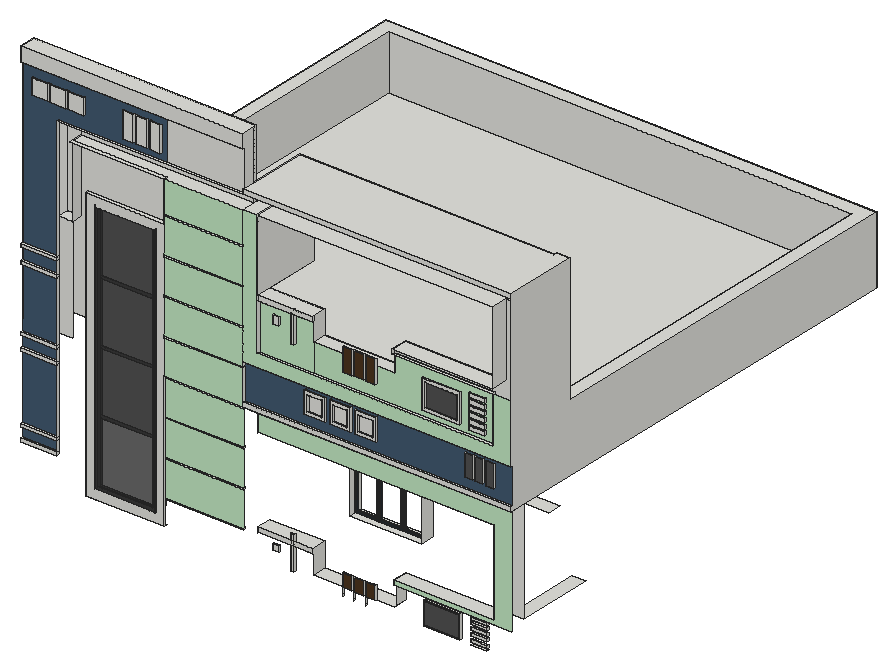
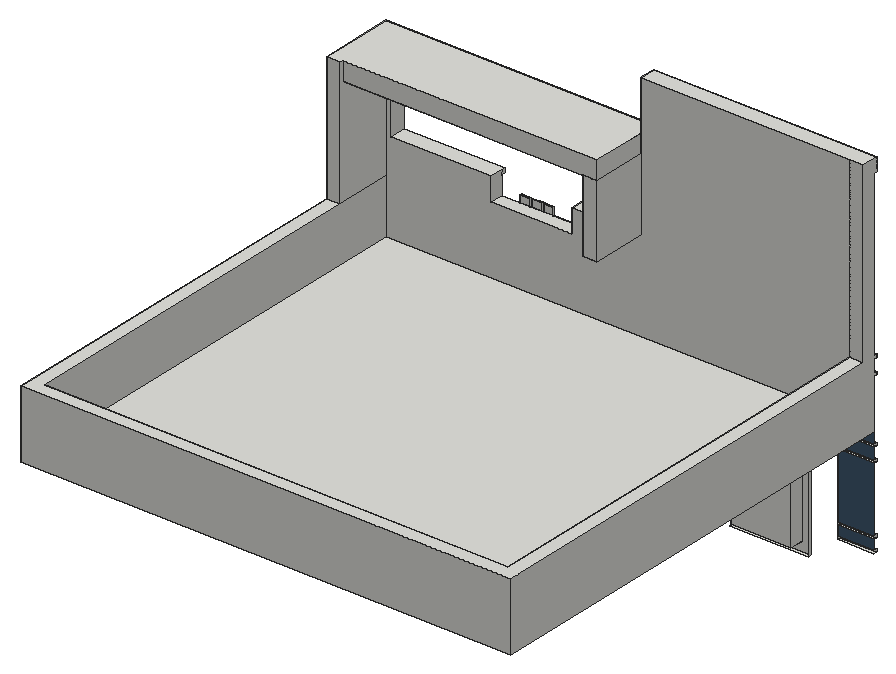
# SketchUp Ruby script. Lengths in inches.
U = 1.inch
M = Sketchup.active_model
def pt(a) = Geom::Point3d.new(a.map { |v| v * U })
def face(e, loops, mat)
  f = e.add_face(loops[0].map { |a| pt(a) })
  loops[1..].each { |l| e.add_face(l.map { |a| pt(a) }).erase! }
  f.material = f.back_material = mat if mat
  f
end
# faces: each face lists its corners as indices into pts; further lists are holes
def faces(e, pts, list, mat = nil) = list.each { |f| face(e, (f[0].is_a?(Array) ? f : [f]).map { |l| l.map { |i| pts[i] } }, mat) }
# xy, xz, yz: faces in a plane at the given z, y or x. An outline is a flat list of corners, or four numbers for a rectangle; further outlines are holes
def ring(l) = l.size == 4 ? [[l[0], l[1]], [l[2], l[1]], [l[2], l[3]], [l[0], l[3]]] : l.each_slice(2).to_a
def flat(e, list, mat, &to3) = list.each { |f| face(e, (f[0].is_a?(Array) ? f : [f]).map { |l| ring(l).map { |u, v| to3.(u, v) } }, mat) }
def xy(e, z, list, mat = nil) = flat(e, list, mat) { |x, y| [x, y, z] }
def xz(e, y, list, mat = nil) = flat(e, list, mat) { |x, z| [x, y, z] }
def yz(e, x, list, mat = nil) = flat(e, list, mat) { |y, z| [x, y, z] }
def lines(e, pts, list) = list.each { |a, b| e.add_line(pt(pts[a]), pt(pts[b])) }
# prism: a flat outline (further loops are holes) pulled along v
def prism(e, loops, v, mat = nil)
  f = face(e, loops, mat); d = Geom::Vector3d.new(v.map { |x| x * U })
  f.pushpull(f.normal.samedirection?(d) ? d.length : -d.length)
end
def box(e, o, s, mat = nil) = prism(e, [[o, [o[0] + s[0], o[1], o[2]], [o[0] + s[0], o[1] + s[1], o[2]], [o[0], o[1] + s[1], o[2]]]], [0, 0, s[2]], mat)
def at(x, y, z, deg = 0) = Geom::Transformation.translation(pt([x, y, z])) * Geom::Transformation.rotation(ORIGIN, Z_AXIS, deg.degrees)
def axes(o, x, y, z) = Geom::Transformation.new([*x, 0, *y, 0, *z, 0, *pt(o).to_a, 1])
def part(name) = M.definitions.add(name)
# library, detail: a bought-in or finely detailed component or shape, given as its bounding box
def library(name, o, s) = part(name).tap { |d| box(d.entities, o, s) }
def detail(e, o, s) = box(e.add_group.entities, o, s)
def put(e, d, t, mat = nil) = e.add_instance(d, t).tap { |i| i.material = mat if mat }
def group(e, t, mat = nil) = e.add_group.tap { |g| g.transformation = t; g.material = mat if mat }.entities
root = M.entities
M.materials.add("Teddy_SkinShadow ").color = [76, 52, 30]
M.materials.add("Wine2").color = [0, 0, 0]
M.materials["Wine2"].alpha = 0
M.materials.add("[0111_SlateGray]").color = [66, 89, 112]
M.materials.add("[0116_Lavender]").color = [195, 232, 195]
M.materials.add("[0130_Gainsboro]").color = [39, 45, 50]
M.materials.add("[0134_DimGray]").color = [105, 105, 105]
M.materials.add("[0135_DarkGray]1").color = [81, 81, 81]
M.materials.add("[0136_Charcoal]").color = [35, 35, 35]
M.materials.add("[Color M07]").color = [58, 58, 58]
c1 = part("Framed glazing panel")
xy(c1.entities,0,[[0,-0.98,43.07,0],[0,0,43.07,1.4]],"[0130_Gainsboro]")
xy(c1.entities,0.3,[[0.3,-1.43,42.77,-0.98]],"[0130_Gainsboro]")
xy(c1.entities,2.95,[[2.95,-1.43,40.12,-0.63],[2.95,-0.63,40.12,0],[2.95,0,40.12,0.64],[2.95,0.64,40.12,1.4]],"[0130_Gainsboro]")
xy(c1.entities,3.54,[[3.54,-0.63,39.53,0],[3.54,0,39.53,0.64]],"[0130_Gainsboro]")
xy(c1.entities,111.8125,[[3.54,-0.63,39.53,0],[3.54,0,39.53,0.64]],"[0130_Gainsboro]")
xy(c1.entities,112.4,[[2.95,-1.43,40.12,-0.63],[2.95,-0.63,40.12,0],[2.95,0,40.12,0.64],[2.95,0.64,40.12,1.4]],"[0130_Gainsboro]")
xy(c1.entities,115.05,[[0.3,-1.43,42.77,-0.98]],"[0130_Gainsboro]")
xy(c1.entities,115.35,[[0,-0.98,43.07,0],[0,0,43.07,1.4]],"[0130_Gainsboro]")
xz(c1.entities,-1.43,[[[0.3,0.3,42.77,115.05],[2.95,2.95,40.12,112.4]]],"[0130_Gainsboro]")
xz(c1.entities,-0.98,[[[0,0,43.07,115.35],[0.3,0.3,42.77,115.05]]],"[0130_Gainsboro]")
xz(c1.entities,-0.63,[[[2.95,2.95,40.12,112.4],[3.54,3.54,39.53,111.8125]]],"[0130_Gainsboro]")
xz(c1.entities,0,[[3.54,3.54,39.53,111.8125]],"Wine2")
xz(c1.entities,0,[[[0,0,43.07,115.35],[2.95,2.95,40.12,112.4]],[[2.95,2.95,40.12,112.4],[3.54,3.54,39.53,111.8125]]],"[0130_Gainsboro]")
xz(c1.entities,0.64,[[[2.95,2.95,40.12,112.4],[3.54,3.54,39.53,111.8125]]],"[0130_Gainsboro]")
xz(c1.entities,1.4,[[[0,0,43.07,115.35],[2.95,2.95,40.12,112.4]]],"[0130_Gainsboro]")
yz(c1.entities,0,[[-0.98,0,0,115.35],[0,0,1.4,115.35]],"[0130_Gainsboro]")
yz(c1.entities,0.3,[[-1.43,0.3,-0.98,115.05]],"[0130_Gainsboro]")
yz(c1.entities,2.95,[[-1.43,2.95,-0.63,112.4],[-0.63,2.95,0,112.4],[0,2.95,0.64,112.4],[0.64,2.95,1.4,112.4]],"[0130_Gainsboro]")
yz(c1.entities,3.54,[[-0.63,3.54,0,111.8125],[0,3.54,0.64,111.8125]],"[0130_Gainsboro]")
yz(c1.entities,39.53,[[-0.63,3.54,0,111.8125],[0,3.54,0.64,111.8125]],"[0130_Gainsboro]")
yz(c1.entities,40.12,[[-1.43,2.95,-0.63,112.4],[-0.63,2.95,0,112.4],[0,2.95,0.64,112.4],[0.64,2.95,1.4,112.4]],"[0130_Gainsboro]")
yz(c1.entities,42.77,[[-1.43,0.3,-0.98,115.05]],"[0130_Gainsboro]")
yz(c1.entities,43.07,[[-0.98,0,0,115.35],[0,0,1.4,115.35]],"[0130_Gainsboro]")
c2 = part("Glazed window assembly")
put(c2.entities,c1,axes([90.57,1.43,0],[1.05148,0,0],[0,1,0],[0,0,1]))
put(c2.entities,c1,axes([0,1.43,0],[1.05148,0,0],[0,1,0],[0,0,1]))
put(c2.entities,c1,axes([45.29,1.43,0],[1.05148,0,0],[0,1,0],[0,0,1]))
c3 = part("window")
g1 = group(c3.entities,at(0,0,0))
g2 = group(g1,at(1.57,1.57,27.56))
yz(g2,0,[[0,0,20.47,25.2]],"[0135_DarkGray]1")
g3 = group(g1,at(1.57,1.57,1.57))
yz(g3,0,[[0,0,20.47,25.2]],"[0134_DimGray]")
g4 = group(g1,at(1.57,1.57,53.54),"[0135_DarkGray]1")
yz(g4,0,[[0,0,20.47,25.2]],"[0135_DarkGray]1")
g5 = group(g1,at(1.57,1.57,79.53))
yz(g5,0,[[0,0,20.47,25.2]],"[0135_DarkGray]1")
g6 = group(g1,at(0,0,0))
xy(g6,0,[[0,0,2.76,23.62]],"[Color M07]")
xy(g6,1.18,[[0,1.18,1.18,22.44],[1.97,1.18,2.76,22.44]],"[Color M07]")
xy(g6,1.57,[[1.18,1.57,1.97,22.05]],"[Color M07]")
xy(g6,26.77,[[1.18,1.57,1.97,22.05]],"[Color M07]")
xy(g6,27.56,[[1.18,1.57,1.97,22.05]],"[Color M07]")
xy(g6,52.76,[[1.18,1.57,1.97,22.05]],"[Color M07]")
xy(g6,53.54,[[1.18,1.57,1.97,22.05]],"[Color M07]")
xy(g6,78.74,[[1.18,1.57,1.97,22.05]],"[Color M07]")
xy(g6,79.53,[[1.18,1.57,1.97,22.05]],"[Color M07]")
xy(g6,104.72,[[1.18,1.57,1.97,22.05]],"[Color M07]")
xy(g6,105.12,[[0,1.18,1.18,22.44],[1.97,1.18,2.76,22.44]],"[Color M07]")
xy(g6,106.3,[[0,0,2.76,23.62]],"[Color M07]")
xz(g6,0,[[0,0,2.76,106.3]],"[Color M07]")
xz(g6,1.18,[[0,1.18,1.18,105.12],[1.97,1.18,2.76,105.12]],"[Color M07]")
xz(g6,1.57,[[1.18,1.57,1.97,26.77],[1.18,27.56,1.97,52.76],[1.18,53.54,1.97,78.74],[1.18,79.53,1.97,104.72]],"[Color M07]")
xz(g6,22.05,[[1.18,1.57,1.97,26.77],[1.18,27.56,1.97,52.76],[1.18,53.54,1.97,78.74],[1.18,79.53,1.97,104.72]],"[Color M07]")
xz(g6,22.44,[[0,1.18,1.18,105.12],[1.97,1.18,2.76,105.12]],"[Color M07]")
xz(g6,23.62,[[0,0,2.76,106.3]],"[Color M07]")
yz(g6,0,[[[0,0,23.62,106.3],[1.18,1.18,22.44,105.12]]],"[Color M07]")
yz(g6,1.18,[[[1.18,1.18,22.44,105.12],[1.57,79.53,22.05,104.72],[1.57,53.54,22.05,78.74],[1.57,1.57,22.05,26.77],[1.57,27.56,22.05,52.76]]],"[Color M07]")
yz(g6,1.97,[[[1.18,1.18,22.44,105.12],[1.57,79.53,22.05,104.72],[1.57,1.57,22.05,26.77],[1.57,53.54,22.05,78.74],[1.57,27.56,22.05,52.76]]],"[Color M07]")
yz(g6,2.76,[[[0,0,23.62,106.3],[1.18,1.18,22.44,105.12]]],"[Color M07]")
xy(root,159.46,[[330.79,39.75,341.29,40.75]])
xy(root,160.18,[[299.99,39,323.67,40.75]])
xy(root,160.2,[[78.11,37,130.11,39]])
xy(root,160.9,[[330.79,39.75,341.29,40.75]])
xy(root,162.5625,[[212.91,38,215.16,39]])
xy(root,162.65,[[330.79,39.75,341.29,40.75]])
xy(root,164.71,[[330.79,39.75,341.29,40.75]])
xy(root,164.72,[[247.03,38,253.34,39],[254.72,38,261.03,39],[262.4,38,268.72,39],[227.375,39,280.75,48]])
xy(root,165,[[203,99,251,108]])
xy(root,166.2,[[84.11,37,124.11,46]])
xy(root,166.46,[[330.79,39.75,341.29,40.75]])
xy(root,168.15,[[330.79,39.75,341.29,40.75]])
xy(root,169.9,[[330.79,39.75,341.29,40.75]])
xy(root,170.65,[[201.03,38,204.85,39]])
xy(root,171.46,[[330.79,39.75,341.29,40.75]])
xy(root,173.18,[[247.03,38,253.34,39],[254.72,38,261.03,39],[262.4,38,268.72,39]])
xy(root,173.21,[[330.79,39.75,341.29,40.75]])
xy(root,174.4,[[330.79,39.75,341.29,40.75]])
xy(root,174.46,[[201.03,38,204.85,39]])
xy(root,175.49,[[299.99,39,323.67,40.75]])
xy(root,176,[[130.11,37.5,182,39]])
xy(root,176.15,[[330.79,39.75,341.29,40.75]])
xy(root,177,[[130.11,37.5,182,39]])
xy(root,177.03,[[35,37,59,39]])
xy(root,177.875,[[191.375,38,212.91,39],[215.16,38,227.375,39],[280.75,38,347,40.75]])
xy(root,179.03,[[35,37,59,39]])
xy(root,180.875,[[191.375,38,212.91,38,212.91,39,215.16,39,215.16,38,227.375,38,227.375,48,191.375,48],[212.91,38,215.16,39],[280.75,38,347,48],[350,48,359,99]])
xy(root,184.6875,[[212.91,38,215.16,39]])
xy(root,185.53,[[35,37,59,39]])
xy(root,187.53,[[35,37,59,39]])
xy(root,200,[[130.11,37.5,182,39]])
xy(root,201,[[130.11,37.5,182,39]])
xy(root,213,[[203,99,251,108],[287,99,334.8125,108]])
xy(root,224,[[130.11,37.5,182,39]])
xy(root,225,[[130.11,37.5,182,39]])
xy(root,230.47,[[35,37,59,39]])
xy(root,232.47,[[35,37,59,39]])
xy(root,237,[[191.375,38,347,48]])
xy(root,239.9,[[35,37,59,39]])
xy(root,241.9,[[35,37,59,39]])
xy(root,248,[[130.11,37.5,182,39]])
xy(root,249,[[130.11,37,182,39],[182,37,191.375,37.5],[191.375,37,359,38],[191.375,38,359,48],[191.375,48,359,99]])
xy(root,252,[[182,37,191.375,39],[191.375,37,359,39]])
xy(root,258,[[44,48,350,330]])
xy(root,258.375,[[221.83,38,235.58,39],[238.46,38,252.21,39],[255.27,38,269.02,39],[327.94,38,332.88,39],[334.69,38,339.63,39],
  [342,38,346.94,39]])
xy(root,260.375,[[223.83,38,233.58,39],[240.46,38,250.21,39],[257.27,38,267.02,39]])
xy(root,270.6875,[[223.83,38,233.58,39],[240.46,38,250.21,39],[257.27,38,267.02,39]])
xy(root,272,[[130.11,37,182,39]])
xy(root,272.6875,[[221.83,38,235.58,39],[238.46,38,252.21,39],[255.27,38,269.02,39],[327.94,38,332.88,39],[334.69,38,339.63,39],
  [342,38,346.94,39]])
xy(root,273,[[130.11,37,182,39]])
xy(root,276,[[182,37,359,39]])
xy(root,281.97,[[35,37,59,39]])
xy(root,283.97,[[35,37,59,39]])
xy(root,284.25,[[191.375,37,227.375,39],[227.375,37,347,39]])
xy(root,287.24,[[330.45,38,340.89,39]])
xy(root,288.03,[[299.64,38,324.7,39]])
xy(root,289.86,[[330.45,38,340.89,39]])
xy(root,290.03,[[301.64,38,322.7,39]])
xy(root,290.93,[[330.45,38,340.89,39]])
xy(root,292.22,[[35,37,59,39]])
xy(root,292.4,[[247.03,38,253.34,39],[254.72,38,261.03,39],[262.4,38,268.72,39]])
xy(root,293.55,[[330.45,38,340.89,39]])
xy(root,294,[[35,48,44,48,44,330,350,330,350,86,359,86,359,339,35,339]])
xy(root,294.22,[[35,37,59,39]])
xy(root,295.05,[[330.45,38,340.89,39]])
xy(root,296,[[130.11,37,182,39]])
xy(root,296.97,[[212.91,38,215.16,39]])
xy(root,297,[[130.11,37,182,39]])
xy(root,297.68,[[330.45,38,340.89,39]])
xy(root,299.05,[[330.45,38,340.89,39]])
xy(root,301.68,[[330.45,38,340.89,39]])
xy(root,302.74,[[330.45,38,340.89,39]])
xy(root,302.75,[[227.375,39,280.59,48]])
xy(root,304.5625,[[201.03,38,204.85,39]])
xy(root,305.36,[[330.45,38,340.89,39]])
xy(root,305.47,[[301.64,38,322.7,39]])
xy(root,306.68,[[330.45,38,340.89,39]])
xy(root,307.3125,[[247.03,38,253.34,39],[254.72,38,261.03,39],[262.4,38,268.72,39]])
xy(root,307.47,[[299.64,38,324.7,39]])
xy(root,309.3,[[330.45,38,340.89,39]])
xy(root,309.82,[[201.03,38,204.85,39]])
xy(root,315,[[280.59,37,347,39],[191.375,38,212.91,39],[215.16,38,227.375,39]])
xy(root,318,[[280.59,37,347,48],[191.375,38,212.91,38,212.91,39,215.16,39,215.16,38,227.375,38,227.375,48,191.375,48],[59,39,68,46],[182,48,191,84],[191,48,191.375,84]])
xy(root,320,[[130.11,37,182,39]])
xy(root,321,[[130.11,37,182,39]])
xy(root,333.39,[[84.11,37,124.11,46]])
xy(root,339.39,[[78.11,37,130.11,39]])
xy(root,344,[[130.11,37,182,39]])
xy(root,345,[[130.11,37,182,39]])
xy(root,366,[[130.11,37,182,37,182,46,68,46,68,39,130.11,39],[68,37,130.11,39],[182,37,191.375,84],[191.375,37,347,84],[347,48,350,84]])
xy(root,375,[[59,37,182,39]])
xy(root,378,[[182,37,359,37,359,86,350,86,350,84,182,84]])
xy(root,379.21,[[101.7,38,108.82,39],[110.64,38,117.76,39],[119.57,38,126.7,39]])
xy(root,383.95,[[41.71,38,52.15,39],[53.59,38,64.03,39],[65.46,38,75.9,39]])
xy(root,394.38,[[41.71,38,52.15,39],[53.59,38,64.03,39],[65.46,38,75.9,39]])
xy(root,396.03,[[101.7,38,108.82,39],[110.64,38,117.76,39],[119.57,38,126.7,39]])
xy(root,402,[[35,37,130.11,39],[130.11,37,182,39]])
xy(root,411,[[35,37,182,48]])
xz(root,37,[[[78.11,160.2,130.11,339.39],[84.11,166.2,124.11,333.39]],[35,177.03,59,179.03],[35,185.53,59,187.53],[35,230.47,59,232.47],[35,239.9,59,241.9],
  [182,249,359,252],[35,281.97,59,283.97],[35,292.22,59,294.22],[182,375,359,378],[35,402,182,411]])
xz(root,37,[[130.11,249,182,272],[130.11,273,182,296],[182,276,359,276,359,315,347,315,347,284.25,191.375,284.25,191.375,366,182,366],[130.11,297,182,320],[130.11,321,182,344],
  [130.11,345,182,366]],"[0116_Lavender]")
xz(root,37.5,[[130.11,177,182,200],[130.11,201,182,224],[130.11,225,182,248]],"[0116_Lavender]")
xz(root,38,[[212.91,162.5625,215.16,177.875],[201.03,170.65,204.85,174.46],[191.375,177.875,212.91,180.875],[212.91,177.875,215.16,180.875],[215.16,177.875,227.375,180.875],
  [212.91,180.875,215.16,184.6875],[[221.83,258.375,235.58,272.6875],[223.83,260.375,233.58,270.6875]],[[238.46,258.375,252.21,272.6875],[240.46,260.375,250.21,270.6875]],[[255.27,258.375,269.02,272.6875],[257.27,260.375,267.02,270.6875]],[330.45,287.24,340.89,289.86],
  [[299.64,288.03,324.7,307.47],[301.64,290.03,322.7,305.47]],[330.45,290.93,340.89,293.55],[330.45,295.05,340.89,297.68],[212.91,296.97,215.16,315],[330.45,299.05,340.89,301.68],
  [330.45,302.74,340.89,305.36],[201.03,304.5625,204.85,309.82],[330.45,306.68,340.89,309.3],[191.375,315,227.375,318],[101.7,379.21,108.82,396.03],
  [110.64,379.21,117.76,396.03],[119.57,379.21,126.7,396.03],[41.71,383.95,52.15,394.38],[53.59,383.95,64.03,394.38],[65.46,383.95,75.9,394.38]])
xz(root,38,[[247.03,164.72,253.34,173.18],[254.72,164.72,261.03,173.18],[262.4,164.72,268.72,173.18],[247.03,292.4,253.34,307.3125],[254.72,292.4,261.03,307.3125],
  [262.4,292.4,268.72,307.3125]],"Teddy_SkinShadow ")
xz(root,38,[[280.75,177.875,359,177.875,359,249,191.375,249,191.375,237,347,237,347,180.875,280.75,180.875]],"[0116_Lavender]")
xz(root,38,[[327.94,258.375,332.88,272.6875],[334.69,258.375,339.63,272.6875],[342,258.375,346.94,272.6875]],"[0135_DarkGray]1")
xz(root,39,[[247.03,164.72,253.34,173.18],[254.72,164.72,261.03,173.18],[262.4,164.72,268.72,173.18],[130.11,176,182,177],[212.91,180.875,215.16,184.6875],
  [130.11,200,182,201],[130.11,224,182,225],[130.11,248,182,249],[59,249,68,318],[223.83,260.375,233.58,270.6875],
  [240.46,260.375,250.21,270.6875],[257.27,260.375,267.02,270.6875],[130.11,272,182,273],[254.72,292.4,261.03,302.75],[262.4,292.4,268.72,302.75],
  [130.11,296,182,297],[247.03,302.75,253.34,307.3125],[254.72,302.75,261.03,307.3125],[262.4,302.75,268.72,307.3125],[130.11,320,182,321],
  [130.11,344,182,345],[130.11,375,182,402]])
xz(root,39,[[35,179.03,59,185.53],[35,187.53,59,230.47],[35,232.47,59,239.9],[35,241.9,59,281.97],[[182,252,359,276],[221.83,258.375,235.58,272.6875],[238.46,258.375,252.21,272.6875],[255.27,258.375,269.02,272.6875],[327.94,258.375,332.88,272.6875],[334.69,258.375,339.63,272.6875],[342,258.375,346.94,272.6875]],
  [35,283.97,59,292.22],[[35,294.22,59,294.22,59,375,130.11,375,130.11,402,35,402],[119.57,379.21,126.7,396.03],[110.64,379.21,117.76,396.03],[101.7,379.21,108.82,396.03],[65.46,383.95,75.9,394.38],[53.59,383.95,64.03,394.38],[41.71,383.95,52.15,394.38]]],"[0111_SlateGray]")
xz(root,39,[[[191.375,284.25,227.375,284.25,227.375,315,215.16,315,215.16,296.97,212.91,296.97,212.91,315,191.375,315],[201.03,304.5625,204.85,309.82]],[[227.375,284.25,347,284.25,347,315,280.59,315,280.59,302.75,268.72,302.75,268.72,292.4,262.4,292.4,262.4,302.75,261.03,302.75,261.03,292.4,254.72,292.4,254.72,302.75,253.34,302.75,253.34,292.4,247.03,292.4,247.03,302.75,227.375,302.75],[299.64,288.03,324.7,307.47],[330.45,287.24,340.89,289.86],[330.45,290.93,340.89,293.55],[330.45,295.05,340.89,297.68],[330.45,299.05,340.89,301.68],[330.45,302.74,340.89,305.36],[330.45,306.68,340.89,309.3]]],"[0116_Lavender]")
xz(root,39,[[300.99,161.18,322.67,174.49],[301.64,290.03,322.7,305.47]],"[0135_DarkGray]1")
xz(root,39,[[[299.99,160.18,323.67,175.49],[300.99,161.18,322.67,174.49]]],"[0136_Charcoal]")
xz(root,39.75,[[330.79,160.9,341.29,162.65],[330.79,164.71,341.29,166.46],[330.79,168.15,341.29,169.9],[330.79,171.46,341.29,173.21],[330.79,174.4,341.29,176.15]])
xz(root,46,[[84.11,166.2,124.11,333.39]])
xz(root,48,[[350,180.875,359,249],[44,258,44,411,182,411,182,318,227.375,318,227.375,302.75,280.59,302.75,280.59,318,347,318,347,366,350,366,350,258],[35,294,44,411]])
xz(root,84,[[182,318,191.375,366],[182,366,350,378]])
xz(root,86,[[350,294,359,378]])
xz(root,330,[[44,258,350,294]])
xz(root,339,[[35,249,359,294]])
yz(root,35,[[39,249,39,281.97,37,281.97,37,283.97,39,283.97,39,292.22,37,292.22,37,294.22,39,294.22,39,402,37,402,37,411,48,411,48,294,339,294,339,249]])
yz(root,41.71,[[38,383.95,39,394.38]])
yz(root,44,[[48,258,330,294]])
yz(root,52.15,[[38,383.95,39,394.38]])
yz(root,53.59,[[38,383.95,39,394.38]])
yz(root,59,[[37,177.03,39,179.03],[37,179.03,39,185.53],[37,185.53,39,187.53],[37,187.53,39,230.47],[37,230.47,39,232.47],
  [37,232.47,39,239.9],[37,239.9,39,241.9],[37,241.9,39,281.97],[37,281.97,39,283.97],[37,283.97,39,292.22],
  [37,292.22,39,294.22],[37,294.22,39,375]])
yz(root,64.03,[[38,383.95,39,394.38]])
yz(root,65.46,[[38,383.95,39,394.38]])
yz(root,68,[[39,318,46,366]])
yz(root,75.9,[[38,383.95,39,394.38]])
yz(root,78.11,[[37,160.2,39,339.39]])
yz(root,84.11,[[37,166.2,46,333.39]])
yz(root,101.7,[[38,379.21,39,396.03]])
yz(root,108.82,[[38,379.21,39,396.03]])
yz(root,110.64,[[38,379.21,39,396.03]])
yz(root,117.76,[[38,379.21,39,396.03]])
yz(root,119.57,[[38,379.21,39,396.03]])
yz(root,124.11,[[37,166.2,46,333.39]])
yz(root,126.7,[[38,379.21,39,396.03]])
yz(root,130.11,[[37,160.2,37.5,160.2,37.5,176,39,176,39,177,37.5,177,37.5,200,39,200,39,201,37.5,201,37.5,224,39,224,39,225,37.5,225,37.5,248,39,248,39,249,37,249],[37,272,39,273],[37,296,39,297],[37,320,39,321],[37,339.39,39,344],
  [37,345,39,366]])
yz(root,182,[[37.5,176,39,177],[37.5,200,39,201],[37.5,224,39,225],[37.5,248,39,249],[37,252,39,272],
  [37,273,39,276],[37,296,39,297],[48,318,84,366],[37,320,39,321],[37,344,39,345],
  [46,366,48,378],[48,366,84,378],[37,375,39,378],[39,378,46,378,46,411,37,411,37,402,39,402],[46,378,48,411]])
yz(root,191.375,[[37.5,177.875,38,180.875],[37.5,237,38,249],[38,237,48,249],[48,237,49.5,249],[37,284.25,39,315],
  [37,315,38,366],[38,318,84,366]])
yz(root,201.03,[[38,170.65,39,174.46],[38,304.5625,39,309.82]])
yz(root,203,[[99,165,108,213]])
yz(root,204.85,[[38,170.65,39,174.46],[38,304.5625,39,309.82]])
yz(root,212.91,[[38,162.5625,39,177.875],[38,180.875,39,184.6875],[38,296.97,39,315]])
yz(root,215.16,[[38,162.5625,39,177.875],[38,180.875,39,184.6875],[38,296.97,39,315]])
yz(root,221.83,[[38,258.375,39,272.6875]])
yz(root,223.83,[[38,260.375,39,270.6875]])
yz(root,227.375,[[39,164.72,48,164.72,48,180.875,38,180.875,38,177.875,39,177.875],[39,302.75,48,318],[38,315,39,318]])
yz(root,233.58,[[38,260.375,39,270.6875]])
yz(root,235.58,[[38,258.375,39,272.6875]])
yz(root,238.46,[[38,258.375,39,272.6875]])
yz(root,240.46,[[38,260.375,39,270.6875]])
yz(root,247.03,[[38,159.43,39,160.68],[38,160.68,39,164.72],[38,164.72,39,173.18],[38,292.4,39,307.3125]])
yz(root,250.21,[[38,260.375,39,270.6875]])
yz(root,251,[[99,165,108,213]])
yz(root,252.21,[[38,258.375,39,272.6875]])
yz(root,253.34,[[38,164.72,39,173.18],[38,292.4,39,307.3125]])
yz(root,254.72,[[38,159.43,39,160.68],[38,160.68,39,164.72],[38,164.72,39,173.18],[38,292.4,39,307.3125]])
yz(root,255.27,[[38,258.375,39,272.6875]])
yz(root,257.27,[[38,260.375,39,270.6875]])
yz(root,261.03,[[38,164.72,39,173.18],[38,292.4,39,307.3125]])
yz(root,262.4,[[38,159.43,39,160.68],[38,160.68,39,164.72],[38,164.72,39,173.18],[38,292.4,39,307.3125]])
yz(root,267.02,[[38,260.375,39,270.6875]])
yz(root,268.72,[[38,164.72,39,173.18],[38,292.4,39,307.3125]])
yz(root,269.02,[[38,258.375,39,272.6875]])
yz(root,280.59,[[39,302.75,48,318],[37,315,39,318]])
yz(root,280.75,[[40.75,164.72,40.75,177.875,38,177.875,38,180.875,48,180.875,48,164.72]])
yz(root,299.64,[[38,288.03,39,307.47]])
yz(root,299.99,[[39,160.18,40.75,175.49]])
yz(root,301.64,[[38,290.03,39,305.47]])
yz(root,322.7,[[38,290.03,39,305.47]])
yz(root,323.67,[[39,160.18,40.75,175.49]])
yz(root,324.7,[[38,288.03,39,307.47]])
yz(root,327.94,[[38,258.375,39,272.6875]])
yz(root,330.45,[[38,287.24,39,289.86],[38,290.93,39,293.55],[38,295.05,39,297.68],[38,299.05,39,301.68],[38,302.74,39,305.36],
  [38,306.68,39,309.3]])
yz(root,330.79,[[39.75,160.9,40.75,162.65],[39.75,164.71,40.75,166.46],[39.75,168.15,40.75,169.9],[39.75,171.46,40.75,173.21],[39.75,174.4,40.75,176.15]])
yz(root,332.88,[[38,258.375,39,272.6875]])
yz(root,334.69,[[38,258.375,39,272.6875]])
yz(root,339.63,[[38,258.375,39,272.6875]])
yz(root,340.89,[[38,287.24,39,289.86],[38,290.93,39,293.55],[38,295.05,39,297.68],[38,299.05,39,301.68],[38,302.74,39,305.36],
  [38,306.68,39,309.3]])
yz(root,341.29,[[39.75,160.9,40.75,162.65],[39.75,164.71,40.75,166.46],[39.75,168.15,40.75,169.9],[39.75,171.46,40.75,173.21],[39.75,174.4,40.75,176.15]])
yz(root,342,[[38,258.375,39,272.6875]])
yz(root,346.94,[[38,258.375,39,272.6875]])
yz(root,347,[[38,180.875,48,237],[37,284.25,39,315],[37,318,48,366]])
yz(root,350,[[48,258,330,294],[48,294,48,366,84,366,84,378,86,378,86,294]])
yz(root,359,[[37,249,339,249,339,294,86,294,86,378,37,378,37,276,39,276,39,252,37,252]])
p = [[59,46,318],[59,46,378],[68,46,366],[68,46,378]]
lines(root,p,[[0,1],[2,3]])
put(root,c2,axes([202.89,103.5,164.875],[0.34927,0,0],[0,0.3234,0],[0,0,0.41611]))
put(root,c3,axes([84.11,41.76,166.2],[0,-1.59,0],[1.7013,0,0],[0,0,1.59]))
